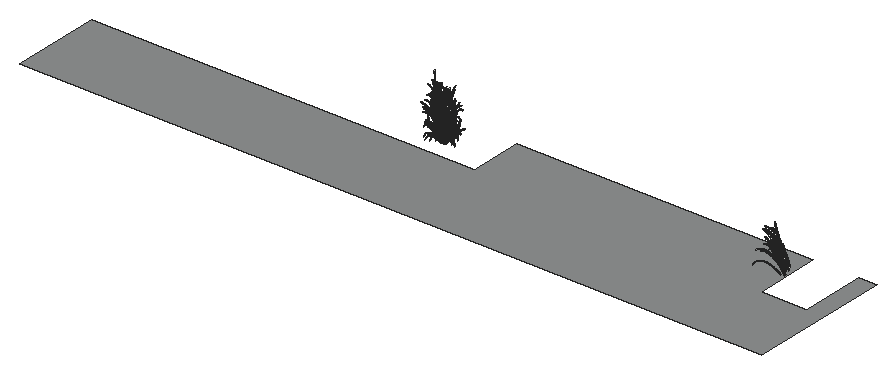
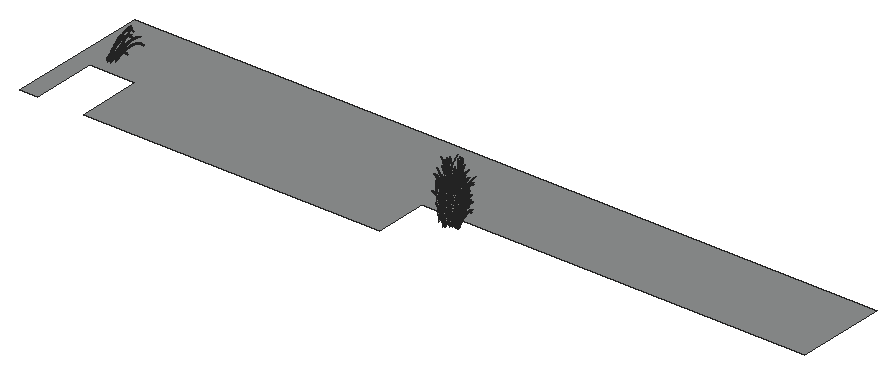
# SketchUp Ruby script. Lengths in inches.
U = 1.inch
M = Sketchup.active_model
def pt(a) = Geom::Point3d.new(a.map { |v| v * U })
def face(e, loops, mat)
  f = e.add_face(loops[0].map { |a| pt(a) })
  loops[1..].each { |l| e.add_face(l.map { |a| pt(a) }).erase! }
  f.material = f.back_material = mat if mat
  f
end
# faces: each face lists its corners as indices into pts; further lists are holes
def faces(e, pts, list, mat = nil) = list.each { |f| face(e, (f[0].is_a?(Array) ? f : [f]).map { |l| l.map { |i| pts[i] } }, mat) }
# xy, xz, yz: faces in a plane at the given z, y or x. An outline is a flat list of corners, or four numbers for a rectangle; further outlines are holes
def ring(l) = l.size == 4 ? [[l[0], l[1]], [l[2], l[1]], [l[2], l[3]], [l[0], l[3]]] : l.each_slice(2).to_a
def flat(e, list, mat, &to3) = list.each { |f| face(e, (f[0].is_a?(Array) ? f : [f]).map { |l| ring(l).map { |u, v| to3.(u, v) } }, mat) }
def xy(e, z, list, mat = nil) = flat(e, list, mat) { |x, y| [x, y, z] }
def xz(e, y, list, mat = nil) = flat(e, list, mat) { |x, z| [x, y, z] }
def yz(e, x, list, mat = nil) = flat(e, list, mat) { |y, z| [x, y, z] }
def lines(e, pts, list) = list.each { |a, b| e.add_line(pt(pts[a]), pt(pts[b])) }
# prism: a flat outline (further loops are holes) pulled along v
def prism(e, loops, v, mat = nil)
  f = face(e, loops, mat); d = Geom::Vector3d.new(v.map { |x| x * U })
  f.pushpull(f.normal.samedirection?(d) ? d.length : -d.length)
end
def box(e, o, s, mat = nil) = prism(e, [[o, [o[0] + s[0], o[1], o[2]], [o[0] + s[0], o[1] + s[1], o[2]], [o[0], o[1] + s[1], o[2]]]], [0, 0, s[2]], mat)
def at(x, y, z, deg = 0) = Geom::Transformation.translation(pt([x, y, z])) * Geom::Transformation.rotation(ORIGIN, Z_AXIS, deg.degrees)
def axes(o, x, y, z) = Geom::Transformation.new([*x, 0, *y, 0, *z, 0, *pt(o).to_a, 1])
def part(name) = M.definitions.add(name)
# library, detail: a bought-in or finely detailed component or shape, given as its bounding box
def library(name, o, s) = part(name).tap { |d| box(d.entities, o, s) }
def detail(e, o, s) = box(e.add_group.entities, o, s)
def put(e, d, t, mat = nil) = e.add_instance(d, t).tap { |i| i.material = mat if mat }
def group(e, t, mat = nil) = e.add_group.tap { |g| g.transformation = t; g.material = mat if mat }.entities
root = M.entities
M.materials.add("[Blacktop Old 02]").color = [143, 145, 145]
c1 = part("fur_instance\#8")
p = [[-0.25,1.49,0.03],[0.25,-1.49,-0.03],[0.44,-1.47,1.51],[-0.05,1.47,1.57],[0.65,-1.44,3.05],[0.16,1.45,3.11],
  [0.86,-1.42,4.59],[0.38,1.44,4.65],[1.1,-1.39,6.13],[0.62,1.43,6.18],[1.34,-1.35,7.66],[0.875,1.42,7.72],
  [1.6,-1.32,9.19],[1.14,1.41,9.25],[1.88,-1.28,10.72],[1.43,1.41,10.78],[2.18,-1.24,12.25],[1.73,1.41,12.3],
  [2.49,-1.19,13.77],[2.05,1.41,13.82],[2.83,-1.15,15.29],[2.4,1.41,15.34],[3.18,-1.09,16.8],[2.76,1.42,16.85],
  [3.56,-1.03,18.31],[3.14,1.43,18.35],[3.96,-0.97,19.81],[3.55,1.44,19.85],[4.38,-0.91,21.3],[3.99,1.46,21.35],
  [4.84,-0.83,22.78],[4.45,1.48,22.83],[5.32,-0.76,24.26],[4.93,1.51,24.31],[5.82,-0.67,25.73],[5.45,1.54,25.77],
  [6.36,-0.59,27.18],[6,1.57,27.23],[6.93,-0.49,28.625],[6.58,1.61,28.67],[7.54,-0.39,30.05],[7.19,1.66,30.1],
  [8.18,-0.28,31.47],[7.84,1.71,31.51],[8.85,-0.16,32.86],[8.53,1.77,32.9],[9.57,-0.04,34.24],[9.25,1.83,34.27],
  [10.32,0.09,35.59],[10.02,1.9,35.625],[11.12,0.23,36.92],[10.82,1.97,36.95],[11.95,0.38,38.22],[11.67,2.06,38.25],
  [12.84,0.54,39.49],[12.57,2.14,39.52],[13.76,0.71,40.73],[13.51,2.24,40.76],[14.73,0.89,41.93],[14.49,2.34,41.95],
  [15.75,1.08,43.09],[15.52,2.45,43.11],[16.82,1.28,44.2],[16.6,2.5625,44.23],[17.93,1.5,45.27],[17.73,2.68,45.29],
  [19.08,1.73,46.28],[18.9,2.81,46.3],[20.29,1.97,47.24],[20.125,2.93,47.26],[21.53,2.22,48.13],[21.39,3.0625,48.15],
  [22.82,2.5,48.96],[22.7,3.1875,48.98],[24.14,2.8125,49.72],[24.06,3.3,49.73],[25.48,3.27,50.41]]
faces(c1.entities,p,[[0,1,2,3],[3,2,4,5],[5,4,6,7],[7,6,8,9],[9,8,10,11],[11,10,12,13],[13,12,14,15],[15,14,16,17],
  [17,16,18,19],[19,18,20,21],[21,20,22,23],[23,22,24,25],[25,24,26,27],[27,26,28,29],[29,28,30,31],[31,30,32,33],
  [33,32,34,35],[35,34,36,37],[37,36,38,39],[39,38,40,41],[41,40,42,43],[43,42,44,45],[45,44,46,47],[47,46,48,49],
  [49,48,50,51],[51,50,52,53],[53,52,54,55],[55,54,56,57],[57,56,58,59],[59,58,60,61],[61,60,62,63],[63,62,64,65],
  [65,64,66,67],[67,66,68,69],[69,68,70,71],[71,70,72,73],[73,72,74,75],[75,74,76]])
xy(root,0,[[5.25,0,453.6875,0,453.6875,86.15,442.8125,86.15,442.8125,47.02,415.52,47.02,415.52,86.15,236.6875,86.15,236.6875,54.02,5.25,54.02]],"[Blacktop Old 02]")
put(root,c1,axes([207.21,65.46,4.97],[0.0229,-0.1484,-0.09458],[0.15576,-0.02704,0.16403],[-0.07366,-0.06935,0.33993]))
put(root,c1,axes([207.5,67.02,7.98],[-0.04613,-0.168,-0.12838],[0.20048,-0.07761,0.07112],[-0.05022,-0.08162,0.45074]))
put(root,c1,axes([207.02,66.9375,7.05],[0.01336,-0.18156,-0.05149],[0.1916,-0.02315,0.12623],[-0.05991,-0.05859,0.42926]))
put(root,c1,axes([206.56,65.12,3.3125],[0.13306,-0.03251,0.2141],[-0.03468,0.1366,0.1095],[-0.09265,-0.07326,0.28274]))
put(root,c1,axes([208.0625,65.3,6.55],[-0.14651,-0.09517,-0.11625],[0.13838,-0.13795,-0.08263],[-0.01824,-0.0963,0.42995]))
put(root,c1,axes([208.78,66.82,9.01],[-0.22374,-0.02944,-0.01516],[0.05551,-0.18692,-0.16154],[0.00543,-0.11272,0.49003]))
put(root,c1,axes([207.68,63.75,3.09],[-0.00857,-0.10681,-0.26092],[0.17656,-0.05814,0.06779],[-0.05152,-0.12704,0.31177]))
put(root,c1,axes([206.59,64.66,3.74],[0.14194,0.01295,0.23971],[-0.09799,0.13483,0.13149],[-0.07264,-0.11667,0.31745]))
put(root,c1,axes([207.44,64.1875,3.29],[0.04246,-0.11664,-0.17724],[0.14637,-0.02684,0.16417],[-0.06419,-0.10309,0.2805]))
put(root,c1,axes([208.59,66.82,7.26],[-0.13872,-0.10688,-0.05008],[0.13478,-0.14007,-0.01499],[-0.01621,-0.05768,0.43132]))
put(root,c1,axes([208.23,67.18,7.01],[-0.09202,-0.14419,-0.02135],[0.16494,-0.10399,0.03603],[-0.02333,-0.03794,0.42396]))
put(root,c1,axes([207.42,66.01,4.62],[0.09225,-0.12894,0.11038],[0.10291,0.0771,0.12838],[-0.07903,-0.02356,0.31361]))
put(root,c1,axes([207.56,63.42,1.75],[0.04168,-0.09258,-0.28201],[0.16554,-0.04371,0.15063],[-0.06017,-0.13932,0.24891]))
put(root,c1,axes([206.71,64.72,3.96],[0.15549,-0.01208,0.20833],[-0.06905,0.13306,0.17126],[-0.07165,-0.11508,0.31313]))
put(root,c1,axes([209.1,65.93,7.09],[-0.18618,-0.03996,-0.02577],[0.06509,-0.15689,-0.1364],[0.00464,-0.09644,0.41925]))
put(root,c1,axes([209.1,65.55,5.67],[-0.15853,0.06077,0.01255],[-0.05151,-0.13731,-0.04414],[-0.00488,-0.05314,0.37046]))
put(root,c1,axes([209.52,64.09,5.28],[-0.25079,-0.01126,0.01167],[0.02691,-0.14432,-0.37072],[0.02191,-0.19373,0.42855]))
put(root,c1,axes([208.99,63.75,3.77],[-0.15193,-0.01941,-0.09588],[0.0644,-0.09304,-0.22233],[-0.00624,-0.12588,0.27933]))
put(root,c1,axes([209.28,62.98,1.5],[-0.16406,0.03446,0.0684],[-0.03839,-0.06194,-0.29017],[-0.00638,-0.14462,0.2315]))
put(root,c1,axes([206.38,63.98,2.34],[0.18766,-0.05407,0.15304],[-0.0375,0.10124,0.3241],[-0.06745,-0.15619,0.27904]))
put(root,c1,axes([208.08,65.78,8.46],[-0.04308,0.17847,0.273],[-0.24701,-0.00413,-0.05166],[-0.00912,-0.15991,0.48813]))
put(root,c1,axes([207.45,64.11,4.21],[0.03417,-0.12525,-0.29157],[0.20378,-0.0224,0.09589],[-0.03382,-0.15429,0.3542]))
put(root,c1,axes([207.74,64.54,5.55],[0.00591,-0.15376,-0.2335],[0.21361,-0.03099,0.04882],[-0.02765,-0.13326,0.41924]))
put(root,c1,axes([208.54,64.44,5.5],[-0.06192,0.14505,0.21697],[-0.19671,-0.02273,-0.07174],[-0.0075,-0.13152,0.40147]))
put(root,c1,axes([209.78,63.75,4.18],[-0.22603,-0.01056,0.00948],[0.02497,-0.13008,-0.33426],[0.01976,-0.17466,0.38636]))
put(root,c1,axes([208.3,65.36,6.98],[0.0038,0.14954,0.23139],[-0.20994,0.03733,-0.03743],[-0.02717,-0.13094,0.41195]))
put(root,c1,axes([208.4,65.625,5.18],[-0.04654,-0.13259,-0.03011],[0.14978,-0.05997,0.02545],[-0.01873,-0.03986,0.3514]))
put(root,c1,axes([208.44,63.08,1.48],[-0.02123,-0.06781,-0.31584],[0.17417,-0.05199,-0.00113],[-0.03366,-0.14772,0.24534]))
put(root,c1,axes([209.32,64.51,6.24],[-0.18897,-0.07724,-0.16578],[0.14014,-0.11074,-0.30364],[0.02044,-0.18069,0.39971]))
put(root,c1,axes([208.47,65.26,6.49],[-0.0211,0.16438,0.13367],[-0.19675,0.00758,-0.04177],[-0.01791,-0.09455,0.42215]))
put(root,c1,axes([209.14,66.02,6.79],[-0.1296,-0.11177,-0.03307],[0.13714,-0.12794,-0.0397],[-0.00189,-0.06022,0.41924]))
put(root,c1,axes([207.97,63.68,2.85],[0.0606,-0.10906,-0.18612],[0.14677,-0.00638,0.15494],[-0.04628,-0.11412,0.28007]))
put(root,c1,axes([209.56,65.31,7.4],[-0.15736,0.12863,0.21317],[-0.17096,-0.10355,-0.14422],[0.01307,-0.14881,0.45294]))
put(root,c1,axes([209.5,64.49,5.2],[-0.16225,-0.04777,-0.05886],[0.07812,-0.11873,-0.19059],[0.01013,-0.11533,0.35104]))
put(root,c1,axes([209.33,65.42,6.21],[-0.13495,-0.09194,-0.07228],[0.12419,-0.11921,-0.10694],[0.00432,-0.08968,0.38985]))
put(root,c1,axes([208.47,66.05,6.99],[-0.00432,-0.15952,-0.128],[0.19173,-0.03266,0.04648],[-0.02798,-0.08806,0.41192]))
put(root,c1,axes([208,63.94,3.66],[0.10535,0.0488,0.23666],[-0.12967,0.10407,0.09442],[-0.04869,-0.12008,0.29468]))
put(root,c1,axes([208.47,66.96,6.43],[-0.00822,-0.16722,0.01164],[0.17876,-0.02595,0.03382],[-0.01925,-0.0303,0.40131]))
put(root,c1,axes([209.61,64.4,4.66],[-0.14242,0.06423,0.07833],[-0.06984,-0.11466,-0.07925],[0.01251,-0.07634,0.33832]))
put(root,c1,axes([209.66,64.98,6.03],[-0.1422,0.11091,0.11586],[-0.12628,-0.11191,-0.06649],[0.015,-0.09153,0.40561]))
put(root,c1,axes([209.92,67.46,8.36],[-0.17633,-0.09809,0.01724],[0.1199,-0.16919,-0.04915],[0.01352,-0.05835,0.47546]))
put(root,c1,axes([209.69,63.61,3.54],[-0.13701,0.06738,0.19305],[-0.11347,-0.07671,-0.17654],[0.01546,-0.13663,0.30225]))
put(root,c1,axes([209.67,65.19,5.49],[-0.14765,0.06695,0.09599],[-0.07527,-0.12279,-0.06548],[0.02169,-0.07701,0.35566]))
put(root,c1,axes([210.05,67.52,9.43],[-0.22223,-0.05187,0.06437],[0.06185,-0.19269,-0.14793],[0.04097,-0.1013,0.49904]))
put(root,c1,axes([207.67,66.37,5.93],[0.1666,-0.05285,0.10887],[0.0248,0.15525,0.04679],[-0.05548,-0.04238,0.37888]))
put(root,c1,axes([209.5625,63.07,1.92],[-0.13424,-0.03889,-0.12787],[0.08866,-0.05443,-0.25596],[0.01839,-0.13945,0.22254]))
put(root,c1,axes([208.78,64.55,5.08],[0.0286,0.11518,0.18982],[-0.16763,0.04809,-0.0018],[-0.022,-0.10604,0.33361]))
put(root,c1,axes([208.2,64.7,4.7],[0.09089,0.09523,0.11248],[-0.12952,0.09997,0.00707],[-0.03129,-0.06837,0.34303]))
put(root,c1,axes([208.93,64.97,5.11],[0.0055,0.12915,0.11043],[-0.15799,0.02454,-0.01796],[-0.01431,-0.07554,0.33727]))
put(root,c1,axes([207.21,66.85,7.83],[0.2061,-0.01344,0.1131],[-0.02793,0.18662,0.09605],[-0.05077,-0.08252,0.4557]))
put(root,c1,axes([209.14,63.37,2.85],[-0.02267,0.09523,0.24051],[-0.16406,0.00552,-0.03477],[-0.00627,-0.12634,0.28034]))
put(root,c1,axes([208.02,65.7,5.77],[0.13539,0.06511,0.11886],[-0.10233,0.13809,0.02305],[-0.04143,-0.06734,0.37184]))
put(root,c1,axes([209.86,66.6,6.71],[-0.12883,-0.11449,0.01319],[0.1336,-0.12723,-0.04151],[0.01291,-0.04776,0.41418]))
put(root,c1,axes([208.29,66.85,9.62],[0.02992,-0.20268,-0.17218],[0.24479,0.00013,0.02509],[-0.00825,-0.12029,0.52424]))
put(root,c1,axes([209.89,67.86,7.57],[-0.11995,-0.14094,0.03187],[0.15995,-0.12378,-0.02155],[0.01135,-0.03745,0.44662]))
put(root,c1,axes([209.96,68.1,10.24],[-0.1863,-0.12854,0.00057],[0.15019,-0.16226,-0.16735],[0.0425,-0.10509,0.5177]))
put(root,c1,axes([209.46,66.31,6.08],[-0.07961,-0.13689,0.01423],[0.15313,-0.0843,-0.034],[0.01219,-0.0383,0.38556]))
put(root,c1,axes([209.46,66.73,6.48],[-0.07772,-0.14595,0.01956],[0.16231,-0.0838,-0.0308],[0.01178,-0.03674,0.40206]))
put(root,c1,axes([209.51,66.22,5.7],[-0.07124,-0.13476,0.02236],[0.14958,-0.07747,-0.02272],[0.00941,-0.03103,0.37011]))
put(root,c1,axes([209.24,63.66,3.64],[0.01737,0.09262,0.24572],[-0.16736,0.02852,0.02395],[-0.00637,-0.12835,0.28481]))
put(root,c1,axes([207.6,67.91,10.27],[0.18706,-0.15692,-0.05371],[0.1539,0.13296,0.16341],[-0.03534,-0.11123,0.5203]))
put(root,c1,axes([208.35,64.9375,4.9],[0.13738,0.0414,0.0972],[-0.07592,0.13055,0.05523],[-0.03104,-0.06782,0.34028]))
put(root,c1,axes([209.74,64.96,6.06],[-0.07914,0.12591,0.21103],[-0.17333,-0.05924,-0.02394],[0.02804,-0.12033,0.37519]))
put(root,c1,axes([209.84,64.61,5.43],[-0.10701,-0.11213,-0.12442],[0.15233,-0.07687,-0.16606],[0.02739,-0.11756,0.36656]))
put(root,c1,axes([210.49,64.56,4.8],[-0.16995,0.00239,0.1052],[-0.0155,-0.13112,-0.16118],[0.04006,-0.1041,0.34197]))
put(root,c1,axes([208.33,63.27,2.44],[0.11054,0.06076,0.32124],[-0.18174,0.06569,0.1961],[-0.00805,-0.18258,0.29226]))
put(root,c1,axes([208.83,66.46,8.02],[0.04164,-0.17352,-0.14577],[0.20763,0.01338,0.03275],[-0.00709,-0.10329,0.45016]))
put(root,c1,axes([208.78,63.36,2.71],[0.07036,0.07691,0.22077],[-0.15002,0.05652,0.10186],[-0.00627,-0.1264,0.28049]))
put(root,c1,axes([208.35,65.46,6.11],[0.15043,0.06237,0.10618],[-0.10193,0.14112,0.07332],[-0.02651,-0.08344,0.39031]))
put(root,c1,axes([208.44,64.57,4.85],[0.1599,-0.01285,0.09328],[-0.0299,0.12534,0.15874],[-0.03604,-0.09723,0.32437]))
put(root,c1,axes([210.76,63.47,2.95],[-0.19796,-0.00213,0.19119],[-0.0584,-0.09827,-0.32515],[0.05556,-0.17894,0.29438]))
put(root,c1,axes([209.27,64.5,5.42],[-0.00485,-0.13574,-0.20923],[0.19174,-0.01245,-0.03687],[0.01079,-0.12284,0.3739]))
put(root,c1,axes([208.24,64.14,4.3],[0.16477,0.01322,0.09468],[-0.05646,0.12716,0.16983],[-0.02254,-0.10862,0.34171]))
put(root,c1,axes([210.91,66.57,6.59],[-0.18521,-0.02955,0.11381],[0.03239,-0.17376,-0.06029],[0.05035,-0.05919,0.41626]))
put(root,c1,axes([210.64,64.2,3.87],[-0.14955,-0.02951,0.08847],[0.01953,-0.12021,-0.14832],[0.04773,-0.08667,0.30915]))
put(root,c1,axes([208.62,63.6,3.27],[0.16669,-0.01734,0.08094],[-0.02966,0.10281,0.23812],[-0.02771,-0.12642,0.29024]))
put(root,c1,axes([208.82,63.39,2.97],[0.12347,0.06755,0.21237],[-0.14396,0.08585,0.17984],[-0.00718,-0.14468,0.32104]))
put(root,c1,axes([210.81,65.25,6.875],[-0.16708,-0.12567,-0.06302],[0.15179,-0.11958,-0.24667],[0.05298,-0.1377,0.45233]))
put(root,c1,axes([208.92,67.21,6.375],[0.10751,-0.14401,0.02773],[0.14274,0.0886,-0.01156],[-0.00773,-0.0245,0.39927]))
put(root,c1,axes([210.01,63.22,2.44],[-0.04322,-0.08103,-0.33227],[0.19342,-0.01502,-0.11763],[0.02265,-0.17179,0.27415]))
put(root,c1,axes([210.28,66.19,5.24],[-0.08777,-0.12311,0.07978],[0.13105,-0.09185,-0.0647],[0.04014,-0.02395,0.34954]))
put(root,c1,axes([210.81,64.67,5.74],[-0.14817,-0.12463,-0.07303],[0.15181,-0.10509,-0.22784],[0.04979,-0.1294,0.42509]))
put(root,c1,axes([209.09,64.26,4.62],[0.12885,0.05972,0.11755],[-0.10424,0.10176,0.1411],[-0.00603,-0.1057,0.32265]))
put(root,c1,axes([210.75,63.19,1.56],[-0.14554,-0.04613,0.08103],[0.01279,-0.07284,-0.26823],[0.06295,-0.12513,0.21981]))
put(root,c1,axes([211.01,64.25,4.59],[-0.14966,0.06135,0.2769],[-0.12806,-0.11932,-0.12286],[0.06613,-0.14624,0.35295]))
put(root,c1,axes([210.75,63.18,1.64],[-0.08929,0.05587,0.30832],[-0.15159,-0.06244,-0.09121],[0.04736,-0.15254,0.25094]))
put(root,c1,axes([208.92,65.71,5.67],[0.16373,-0.03857,0.00921],[0.02397,0.14494,0.04432],[-0.01107,-0.05099,0.36849]))
put(root,c1,axes([210.1875,65.56,5.39],[-0.04201,-0.14205,-0.02716],[0.15521,-0.03808,-0.10788],[0.03986,-0.0584,0.35377]))
put(root,c1,axes([209.11,63.04,1.76],[0.15269,-0.07243,-0.24019],[0.13551,0.04613,0.26977],[-0.00773,-0.17522,0.28049]))
put(root,c1,axes([209.16,64.98,5.3],[0.14874,-0.07113,-0.04632],[0.06911,0.1145,0.10604],[-0.00549,-0.08,0.34865]))
put(root,c1,axes([211,65.57,4.8],[-0.14662,-0.03521,0.15792],[0.02351,-0.14317,-0.07806],[0.07228,-0.05609,0.32502]))
put(root,c1,axes([209.04,66.05,6.11],[0.16142,-0.07143,-0.01571],[0.0631,0.13884,0.04506],[-0.00507,-0.05525,0.3852]))
put(root,c1,axes([209.07,67.26,7.48],[0.12208,-0.15013,-0.02869],[0.15272,0.10311,-0.03034],[0.01381,-0.04339,0.43679]))
put(root,c1,axes([211.25,64.5625,5.75],[-0.10088,0.13062,0.3695],[-0.228,-0.07812,-0.04804],[0.0527,-0.18996,0.43195]))
put(root,c1,axes([209.35,63,1.69],[0.1143,0.07759,0.29786],[-0.18253,0.04472,0.24081],[0.02462,-0.18668,0.29791]))
put(root,c1,axes([209.52,65.15,6.22],[0.10618,-0.13596,-0.12929],[0.15853,0.08066,0.0353],[0.01505,-0.09183,0.40695]))
put(root,c1,axes([210.63,64.25,4.92],[-0.04153,-0.12718,-0.27595],[0.20481,-0.00989,-0.14624],[0.04417,-0.15922,0.36205]))
put(root,c1,axes([209.21,63.21,2.53],[0.19045,-0.03751,-0.06848],[0.03839,0.07261,0.33686],[-0.00736,-0.16676,0.26694]))
put(root,c1,axes([209.79,65.09,5.64],[0.0987,0.11897,0.05521],[-0.14378,0.08662,0.10909],[0.02282,-0.08103,0.37425]))
put(root,c1,axes([209.77,66.72,5.8],[0.11708,-0.12342,-0.00631],[0.12225,0.10057,-0.03033],[0.0076,-0.02912,0.37804]))
put(root,c1,axes([209.74,63.2,2.43],[0.10158,-0.06914,-0.32205],[0.1701,0.0448,0.14301],[0.02265,-0.17174,0.27406]))
put(root,c1,axes([210.66,63.58,3.05],[0.00165,-0.10984,-0.26082],[0.18149,0.01453,-0.07449],[0.03836,-0.13829,0.31445]))
put(root,c1,axes([211.97,65.85,6.76],[-0.1604,-0.13739,-0.02167],[0.15059,-0.11716,-0.25101],[0.06963,-0.12643,0.45099]))
put(root,c1,axes([212.65,64.98,5.43],[-0.21667,0.03837,0.29524],[-0.10928,-0.16078,-0.2283],[0.08148,-0.18018,0.43484]))
put(root,c1,axes([209.69,63.9,3.98],[0.15315,-0.04031,-0.07636],[0.04669,0.1064,0.16007],[0.009,-0.10254,0.31211]))
put(root,c1,axes([212.12,64.41,3.65],[-0.18644,-0.03104,0.19118],[-0.0143,-0.14214,-0.22961],[0.08573,-0.13206,0.3504]))
put(root,c1,axes([210.46,65.08,5.45],[0.0438,-0.14683,-0.11127],[0.16937,0.03664,-0.05087],[0.03107,-0.07683,0.37846]))
put(root,c1,axes([212.13,67.99,9.95],[-0.20857,-0.13075,0.08955],[0.12369,-0.16885,-0.26752],[0.09431,-0.12712,0.50956]))
put(root,c1,axes([209.97,65.82,5.36],[0.13914,-0.08385,-0.03496],[0.08075,0.12335,-0.00894],[0.01158,-0.03859,0.35924]))
put(root,c1,axes([211.69,63.78,1.59],[-0.12758,-0.07753,0.0557],[0.04435,-0.06394,-0.27127],[0.08127,-0.11212,0.2187]))
put(root,c1,axes([211.97,64.0625,2.3],[-0.14977,-0.06071,0.14936],[0.00439,-0.0935,-0.26844],[0.09015,-0.12438,0.2426]))
put(root,c1,axes([211.34,64.36,3.39],[-0.08522,-0.11751,-0.02593],[0.11177,-0.04315,-0.23298],[0.08081,-0.09116,0.27707]))
put(root,c1,axes([210.13,63.84,3.77],[0.12624,-0.07118,-0.14847],[0.09892,0.09301,0.09957],[0.0236,-0.10128,0.3158]))
put(root,c1,axes([209.95,65.81,6.13],[0.11075,-0.11944,-0.11937],[0.13443,0.0987,-0.0216],[0.03784,-0.07056,0.38011]))
put(root,c1,axes([209.1875,66.85,9.9],[0.24074,-0.08114,-0.0797],[0.07823,0.19128,0.15934],[0.00596,-0.12377,0.53808]))
put(root,c1,axes([212.98,64.16,3.13],[-0.23798,-0.07441,0.13592],[0.01899,-0.11962,-0.43721],[0.10286,-0.20447,0.35918]))
put(root,c1,axes([211.61,64.73,3.57],[-0.09743,0.06774,0.23139],[-0.09599,-0.11967,0.05358],[0.09249,-0.07723,0.28321]))
put(root,c1,axes([211.26,64.89,5.37],[-0.02184,-0.15888,-0.15748],[0.19236,-0.00034,-0.15603],[0.06127,-0.11125,0.39683]))
put(root,c1,axes([210.05,65.52,5.3125],[0.15222,0.03642,-0.07852],[-0.03946,0.13914,0.07531],[0.03898,-0.05711,0.34597]))
put(root,c1,axes([211.96,65.35,3.41],[-0.11286,0.04976,0.22948],[-0.06771,-0.13658,0.05175],[0.0986,-0.05954,0.28318]))
put(root,c1,axes([210.67,66.85,6.28],[0.07494,-0.15978,-0.03962],[0.16264,0.06715,-0.11216],[0.04856,-0.037,0.39794]))
put(root,c1,axes([212.01,65.16,4.61],[-0.12334,-0.12969,0.01714],[0.11431,-0.07492,-0.27994],[0.09668,-0.10907,0.33149]))
put(root,c1,axes([210.5,63.32,2.45],[0.09702,-0.05494,-0.31246],[0.152,0.06601,0.10474],[0.04854,-0.15634,0.25719]))
put(root,c1,axes([211.64,68.49,9.47],[-0.02329,-0.21903,-0.03429],[0.23378,-0.02287,-0.15724],[0.06291,-0.07396,0.52011]))
put(root,c1,axes([210.43,66.1,4.98],[0.13682,-0.07692,-0.07129],[0.07213,0.1295,-0.07116],[0.03936,-0.02349,0.34277]))
put(root,c1,axes([209.98,63.61,3.85],[0.22137,0.04305,0.07377],[-0.08148,0.12835,0.33894],[0.02049,-0.18118,0.40078]))
put(root,c1,axes([210.38,63.89,3.92],[0.16263,0.05278,0.0273],[-0.0671,0.09353,0.2615],[0.03718,-0.13404,0.3048]))
put(root,c1,axes([210.27,66.0625,5.73],[0.1463,-0.07615,-0.10409],[0.07711,0.13848,-0.04067],[0.04559,-0.04329,0.3674]))
put(root,c1,axes([212.41,66.03,4.17],[-0.14023,0.01888,0.26296],[-0.04453,-0.1614,-0.00292],[0.11023,-0.06656,0.31656]))
put(root,c1,axes([212.28,64.38,2.35],[-0.13012,-0.10057,0.10963],[0.04873,-0.08061,-0.28847],[0.10836,-0.10823,0.24566]))
put(root,c1,axes([210.85,65.97,5.05],[0.10839,-0.11453,-0.08174],[0.11795,0.10157,-0.07097],[0.04416,-0.04194,0.35588]))
put(root,c1,axes([210.65,65.1,6.95],[0.14666,-0.13638,-0.25039],[0.18844,0.10867,0.09026],[0.03514,-0.1508,0.47019]))
put(root,c1,axes([212.6875,66.26,4],[-0.14894,-0.04461,0.24591],[0.01234,-0.15892,-0.10432],[0.11196,-0.06761,0.32156]))
put(root,c1,axes([212.23,68.4,8.6875],[-0.02212,-0.21398,-0.03391],[0.22838,-0.02174,-0.15347],[0.06144,-0.07223,0.50797]))
put(root,c1,axes([210.2,66.9,9.03],[0.23315,0.01342,-0.06471],[-0.02237,0.19719,0.15093],[0.03065,-0.10883,0.50265]))
put(root,c1,axes([210.96,65.17,4.86],[0.10539,0.11766,-0.04264],[-0.11395,0.08648,0.1779],[0.06944,-0.07112,0.33381]))
put(root,c1,axes([212.9,65.09,3.33],[-0.10089,0.09227,0.28247],[-0.13958,-0.12254,0.05217],[0.09902,-0.11171,0.33951]))
put(root,c1,axes([212.29,65.4,5.95],[-0.03936,0.14543,0.30601],[-0.20696,-0.07562,0.14027],[0.09659,-0.14879,0.39477]))
put(root,c1,axes([210.57,63.79,3.74],[0.19476,0.01919,-0.07142],[-0.00771,0.11743,0.2824],[0.0412,-0.14851,0.33769]))
put(root,c1,axes([211.03,68.37,10.66],[0.12423,-0.19532,-0.16493],[0.21975,0.1108,-0.06089],[0.05484,-0.10226,0.55089]))
put(root,c1,axes([211.34,65.86,7.06],[0.10368,0.16194,0.09463],[-0.18699,0.06759,0.22582],[0.06767,-0.12287,0.43828]))
put(root,c1,axes([211.15,63.51,2.01],[0.10797,-0.02278,-0.25368],[0.09924,0.08349,0.12145],[0.06318,-0.1256,0.22064]))
put(root,c1,axes([211.02,64.28,4.37],[0.12346,-0.06874,-0.2664],[0.133,0.10274,0.08323],[0.06093,-0.13474,0.32518]))
put(root,c1,axes([212.11,67.7,8.47],[-0.03736,-0.20284,-0.08426],[0.21276,-0.01244,-0.24024],[0.09664,-0.09898,0.46456]))
put(root,c1,axes([211.23,67.38,9.57],[0.143,-0.17445,-0.17187],[0.20045,0.12222,-0.01071],[0.04373,-0.10813,0.53269]))
put(root,c1,axes([210.99,63.54,2.48],[0.15494,0.00054,-0.15254],[0.03594,0.10834,0.19122],[0.0534,-0.11809,0.285]))
put(root,c1,axes([211.3,65.4,5.71],[0.10826,0.14171,0.01778],[-0.14869,0.07846,0.21324],[0.07154,-0.09642,0.38649]))
put(root,c1,axes([211.96,64.39,3.98],[0.01148,-0.14011,-0.26001],[0.19146,0.05137,-0.16224],[0.08794,-0.13547,0.35942]))
put(root,c1,axes([211.74,64.33,2.75],[0.05454,-0.09644,-0.21571],[0.13016,0.08062,-0.0942],[0.08114,-0.09154,0.27821]))
put(root,c1,axes([211.12,68.5,10.35],[0.15717,-0.16888,-0.16909],[0.19008,0.14007,-0.03029],[0.05359,-0.09991,0.53827]))
put(root,c1,axes([213.02,65.53,3.6875],[-0.06239,0.13265,0.23168],[-0.15342,-0.10065,0.1704],[0.112,-0.09352,0.34293]))
put(root,c1,axes([212.67,67.65,4.85],[-0.06465,-0.16754,0.157],[0.14103,-0.07728,-0.22676],[0.11827,-0.02606,0.33858]))
put(root,c1,axes([210.85,63.45,2.92],[0.19478,-0.02841,-0.30734],[0.1247,0.10642,0.29017],[0.06226,-0.20052,0.32988]))
put(root,c1,axes([211.5,63.57,2.52],[0.10305,-0.05896,-0.3685],[0.16571,0.09891,0.06527],[0.08407,-0.16713,0.29358]))
put(root,c1,axes([211.36,66.04,8.22],[0.19083,0.13184,0.05677],[-0.15811,0.13743,0.27367],[0.05817,-0.15117,0.49659]))
put(root,c1,axes([211.83,65.21,4.67],[0.13121,0.11551,-0.02739],[-0.11587,0.10209,0.2018],[0.06808,-0.09176,0.36783]))
put(root,c1,axes([212.1,66.79,2.6],[0.04832,-0.14518,0.00787],[0.12065,0.04323,-0.22286],[0.09094,-0.00311,0.27632]))
put(root,c1,axes([212.96,64.8125,4.04],[-0.00332,0.15612,0.27725],[-0.2105,-0.04955,0.19049],[0.09652,-0.14869,0.3945]))
put(root,c1,axes([212.08,65.87,3.07],[0.0496,-0.12974,-0.10453],[0.11629,0.07093,-0.20268],[0.09864,-0.03996,0.27723]))
put(root,c1,axes([212.62,66.11,1.875],[-0.03175,-0.14429,0.13902],[0.10175,-0.04851,-0.23869],[0.11949,-0.01479,0.22844]))
put(root,c1,axes([212.97,65.14,2.65],[-0.05491,0.09737,0.28251],[-0.12379,-0.11722,0.16383],[0.12913,-0.0934,0.26231]))
put(root,c1,axes([213.16,65.13,2.47],[-0.0662,0.08995,0.30205],[-0.12202,-0.12772,0.14438],[0.13238,-0.09575,0.2689]))
put(root,c1,axes([214.09,65.6,3.46],[-0.14869,0.01051,0.38769],[-0.10168,-0.16677,-0.09879],[0.14048,-0.14032,0.31849]))
put(root,c1,axes([211.94,64.83,2.98],[0.12216,0.08749,-0.1288],[-0.05725,0.10364,0.19567],[0.09123,-0.07618,0.27934]))
put(root,c1,axes([213.23,65.27,2.55],[-0.06626,-0.1567,-0.04431],[0.12258,-0.00555,-0.33309],[0.13287,-0.09611,0.2699]))
put(root,c1,axes([213.49,66.85,2.07],[-0.09134,-0.12785,0.22656],[0.07697,-0.11104,-0.22116],[0.1384,-0.04262,0.25929]))
put(root,c1,axes([212.68,64.43,2.89],[0.07572,0.13089,0.20219],[-0.15985,-0.01369,0.30106],[0.10643,-0.14683,0.2864]))
put(root,c1,axes([212.07,66.13,5.26],[0.16409,-0.04331,-0.20606],[0.05728,0.16704,-0.00737],[0.08461,-0.06565,0.38043]))
put(root,c1,axes([212.48,66.375,2.1],[0.06266,-0.1249,-0.10853],[0.0861,0.08678,-0.25374],[0.11938,-0.01478,0.22823]))
put(root,c1,axes([212.26,64.99,3.17],[0.14109,0.00407,-0.23949],[0.03377,0.14579,0.07817],[0.0981,-0.08192,0.30039]))
put(root,c1,axes([212.52,65.55,3.76],[0.12005,-0.06141,-0.26447],[0.09556,0.14151,-0.0324],[0.10376,-0.08664,0.31771]))
put(root,c1,axes([212.4,64.79,3.4],[0.16454,0.02683,-0.22071],[0.01929,0.1451,0.16624],[0.09525,-0.10745,0.32659]))
put(root,c1,axes([214.92,65.3,2.04],[-0.15559,-0.16713,0.03304],[0.11706,-0.06849,-0.43118],[0.15185,-0.15167,0.34426]))
put(root,c1,axes([212.86,66.41,2.01],[0.068,-0.12804,-0.12081],[0.08818,0.09434,-0.26208],[0.12484,-0.01545,0.23865]))
put(root,c1,axes([212.3,66.45,6.79],[0.20769,0.04966,-0.15926],[-0.03101,0.17814,0.18526],[0.08167,-0.11008,0.44127]))
put(root,c1,axes([212.89,65.6,2.42],[0.06859,-0.09014,-0.25373],[0.09618,0.12505,-0.16822],[0.12923,-0.06487,0.24688]))
put(root,c1,axes([212.41,64.54,4.58],[0.20792,-0.04098,-0.29203],[0.11115,0.15527,0.21492],[0.07916,-0.17504,0.42246]))
put(root,c1,axes([212.9375,65.61,2.97],[0.12063,-0.06515,-0.25144],[0.08341,0.14829,-0.07405],[0.10987,-0.06634,0.31554]))
put(root,c1,axes([213.11,65.05,4.63],[0.15805,0.15051,0.05502],[-0.15454,0.08321,0.34889],[0.10135,-0.15612,0.41421]))
put(root,c1,axes([213.24,67.2,7.15],[0.20327,-0.05604,-0.25675],[0.08292,0.19878,0.03195],[0.09822,-0.10059,0.47212]))
put(root,c1,axes([214.52,64.87,2.04],[0.10396,-0.07911,-0.43973],[0.18772,0.13868,-0.01375],[0.12911,-0.17813,0.34745]))
put(root,c1,axes([214.9,67.78,4.82],[0.04979,-0.1895,-0.18773],[0.18438,0.09265,-0.2851],[0.14308,-0.0864,0.41092]))
put(root,c1,axes([214,64.82,1.74],[0.1674,0.12348,-0.15342],[-0.05527,0.10723,0.36025],[0.13749,-0.13733,0.3117]))
put(root,c1,axes([423.54,57.89,13.9375],[-0.16665,-0.10839,-0.24928],[0.10528,-0.22,0.26583],[-0.16455,0.00217,0.44452]))
put(root,c1,axes([424.25,55.48,14.64],[-0.08139,0.23064,-0.15312],[-0.1699,-0.05496,-0.32193],[-0.16391,-0.02606,0.43057]))
put(root,c1,axes([425.51,52.52,16.08],[-0.18691,0.1568,-0.23935],[-0.06787,-0.16218,-0.27405],[-0.15492,-0.08418,0.43132]))
put(root,c1,axes([424.86,54.4,14.78],[-0.11905,0.20326,-0.22454],[-0.13951,-0.10936,-0.26462],[-0.15957,-0.02537,0.41917]))
put(root,c1,axes([424.05,52.83,12.73],[-0.02161,-0.16628,-0.28389],[0.16425,-0.14433,0.32408],[-0.18224,-0.08282,0.344]))
put(root,c1,axes([424.11,50.85,10.74],[-0.07933,-0.07892,-0.44402],[0.19255,-0.17562,0.06989],[-0.14788,-0.14983,0.35337]))
put(root,c1,axes([424.74,55.33,13.21],[-0.09014,-0.18111,-0.08882],[0.15594,-0.13199,0.32093],[-0.15035,0.00199,0.40617]))
put(root,c1,axes([425.89,54.81,11.81],[-0.13408,-0.01944,-0.33055],[0.01755,-0.20151,0.16145],[-0.16419,0.01714,0.30229]))
put(root,c1,axes([424.77,54.11,11.3125],[0.01897,-0.21218,0.0586],[0.13531,-0.01729,0.38322],[-0.17657,-0.01268,0.31544]))
put(root,c1,axes([425.36,52.38,11.57],[-0.03242,-0.16161,-0.19656],[0.13271,-0.12456,0.32589],[-0.17032,-0.04313,0.30667]))
put(root,c1,axes([425.8125,55.5,12.39],[-0.06018,0.17755,-0.31983],[-0.13865,-0.10086,-0.20049],[-0.15862,0.04585,0.31318]))
put(root,c1,axes([426.73,51.38,13.82],[-0.17146,0.07712,-0.27655],[0.00216,-0.17859,-0.14821],[-0.13359,-0.07259,0.37194]))
put(root,c1,axes([426.39,51.51,10.69],[-0.07927,0.1771,-0.13212],[-0.09456,-0.05104,-0.31736],[-0.15384,-0.03896,0.27701]))
